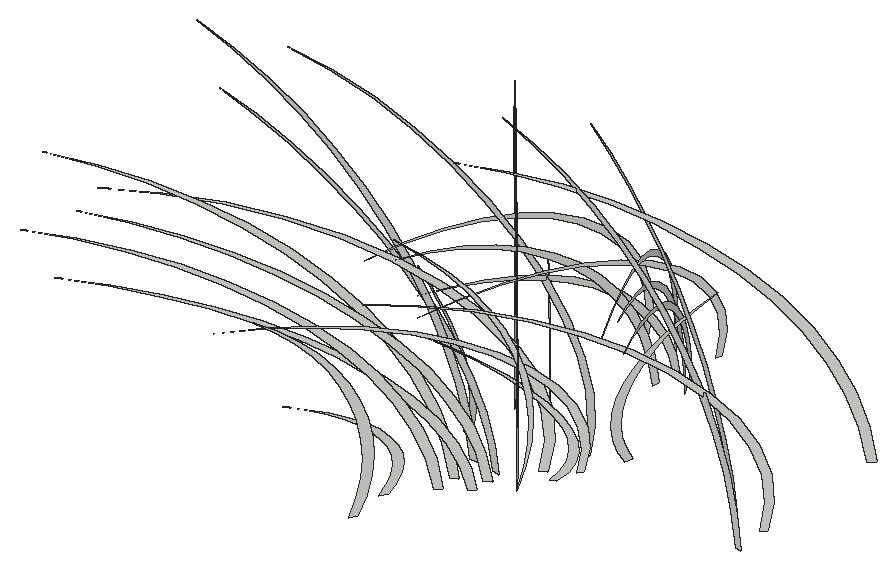
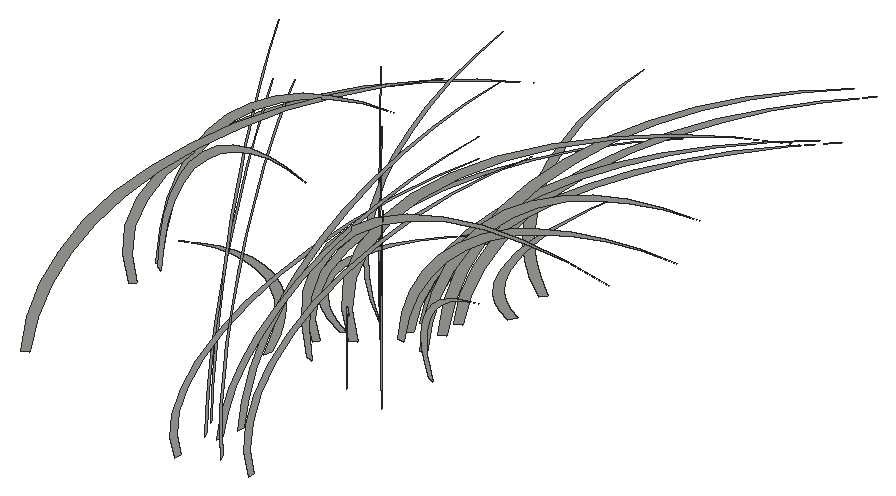
# SketchUp Ruby script. Lengths in inches.
U = 1.inch
M = Sketchup.active_model
def pt(a) = Geom::Point3d.new(a.map { |v| v * U })
def face(e, loops, mat)
  f = e.add_face(loops[0].map { |a| pt(a) })
  loops[1..].each { |l| e.add_face(l.map { |a| pt(a) }).erase! }
  f.material = f.back_material = mat if mat
  f
end
# faces: each face lists its corners as indices into pts; further lists are holes
def faces(e, pts, list, mat = nil) = list.each { |f| face(e, (f[0].is_a?(Array) ? f : [f]).map { |l| l.map { |i| pts[i] } }, mat) }
# xy, xz, yz: faces in a plane at the given z, y or x. An outline is a flat list of corners, or four numbers for a rectangle; further outlines are holes
def ring(l) = l.size == 4 ? [[l[0], l[1]], [l[2], l[1]], [l[2], l[3]], [l[0], l[3]]] : l.each_slice(2).to_a
def flat(e, list, mat, &to3) = list.each { |f| face(e, (f[0].is_a?(Array) ? f : [f]).map { |l| ring(l).map { |u, v| to3.(u, v) } }, mat) }
def xy(e, z, list, mat = nil) = flat(e, list, mat) { |x, y| [x, y, z] }
def xz(e, y, list, mat = nil) = flat(e, list, mat) { |x, z| [x, y, z] }
def yz(e, x, list, mat = nil) = flat(e, list, mat) { |y, z| [x, y, z] }
def lines(e, pts, list) = list.each { |a, b| e.add_line(pt(pts[a]), pt(pts[b])) }
# prism: a flat outline (further loops are holes) pulled along v
def prism(e, loops, v, mat = nil)
  f = face(e, loops, mat); d = Geom::Vector3d.new(v.map { |x| x * U })
  f.pushpull(f.normal.samedirection?(d) ? d.length : -d.length)
end
def box(e, o, s, mat = nil) = prism(e, [[o, [o[0] + s[0], o[1], o[2]], [o[0] + s[0], o[1] + s[1], o[2]], [o[0], o[1] + s[1], o[2]]]], [0, 0, s[2]], mat)
def at(x, y, z, deg = 0) = Geom::Transformation.translation(pt([x, y, z])) * Geom::Transformation.rotation(ORIGIN, Z_AXIS, deg.degrees)
def axes(o, x, y, z) = Geom::Transformation.new([*x, 0, *y, 0, *z, 0, *pt(o).to_a, 1])
def part(name) = M.definitions.add(name)
# library, detail: a bought-in or finely detailed component or shape, given as its bounding box
def library(name, o, s) = part(name).tap { |d| box(d.entities, o, s) }
def detail(e, o, s) = box(e.add_group.entities, o, s)
def put(e, d, t, mat = nil) = e.add_instance(d, t).tap { |i| i.material = mat if mat }
def group(e, t, mat = nil) = e.add_group.tap { |g| g.transformation = t; g.material = mat if mat }.entities
root = M.entities
g1 = group(root,at(13.86,752.1,-58.625))
p = [[-2.41,-3.66,8.31],[-1.97,-2.99,7.78],[-1.57,-2.39,7.2],[-1.22,-1.85,6.58],[-0.92,-1.39,5.92],[-0.67,-1.01,5.22],
  [-0.47,-0.72,4.5],[-0.33,-0.5,3.76],[-0.25,-0.38,3.01],[-0.23,-0.34,2.25],[-0.26,-0.4,1.49],[-0.35,-0.54,0.74],
  [-0.5,-0.77,0],[-0.31,-0.47,0],[-0.14,-0.22,0.75],[-0.04,-0.06,1.51],[0,0,2.29],[-0.03,-0.04,3.0625],
  [-0.12,-0.18,3.83],[-0.27,-0.42,4.58],[-0.49,-0.75,5.31],[-0.77,-1.17,6],[-1.1,-1.68,6.65],[-1.49,-2.27,7.26],
  [-1.93,-2.93,7.82]]
faces(g1,p,[[0,1,2,3,4,5,6,7,8,9,10,11,12,13,14,15,16,17,18,19,20,21,22,23,24]])
g2 = group(root,at(14.625,754.95,-58.625))
p = [[-10.47,-7.14,9.36],[-12.05,-8.22,9.61],[-10.52,-7.17,9.31],[-9.04,-6.16,8.89],[-7.64,-5.2,8.37],[-6.3125,-4.3,7.74],
  [-5.09,-3.47,7.02],[-3.97,-2.71,6.2],[-2.99,-2.04,5.3],[-2.14,-1.46,4.34],[-1.44,-0.98,3.3125],[-0.89,-0.6,2.24],
  [-0.5,-0.34,1.13],[-0.27,-0.1875,0],[0,0,0],[-0.18,-0.125,1.16],[-0.55,-0.375,2.3],[-1.09,-0.74,3.39],
  [-1.8,-1.22,4.44],[-2.66,-1.82,5.43],[-3.68,-2.51,6.34],[-4.83,-3.29,7.15],[-6.1,-4.16,7.875],[-7.48,-5.1,8.49],
  [-8.94,-6.09,8.98]]
faces(g2,p,[[0,1,2,3,4,5,6,7,8,9,10,11,12,13,14,15,16,17,18,19,20,21,22,23,24]])
g3 = group(root,at(15.6,755.62,-58.625))
p = [[-10.47,-7.14,7.55],[-12.05,-8.22,7.75],[-10.52,-7.17,7.51],[-9.04,-6.16,7.17],[-7.64,-5.2,6.75],[-6.3125,-4.3,6.24],
  [-5.09,-3.47,5.66],[-3.97,-2.71,5],[-2.99,-2.04,4.28],[-2.14,-1.46,3.5],[-1.44,-0.98,2.67],[-0.89,-0.6,1.81],
  [-0.5,-0.34,0.91],[-0.27,-0.1875,0],[0,0,0],[-0.18,-0.125,0.93],[-0.55,-0.375,1.85],[-1.09,-0.74,2.74],
  [-1.8,-1.22,3.58],[-2.66,-1.82,4.38],[-3.68,-2.51,5.11],[-4.83,-3.29,5.77],[-6.1,-4.16,6.35],[-7.48,-5.1,6.85],
  [-8.94,-6.09,7.25]]
faces(g3,p,[[0,1,2,3,4,5,6,7,8,9,10,11,12,13,14,15,16,17,18,19,20,21,22,23,24]])
g4 = group(root,at(13.69,753.98,-58.625))
p = [[-2.41,-3.66,4.09],[-1.97,-2.99,3.83],[-1.57,-2.39,3.54],[-1.22,-1.85,3.24],[-0.92,-1.39,2.91],[-0.67,-1.01,2.57],
  [-0.47,-0.72,2.22],[-0.33,-0.5,1.85],[-0.25,-0.38,1.48],[-0.23,-0.34,1.11],[-0.26,-0.4,0.73],[-0.35,-0.54,0.36],
  [-0.5,-0.77,0],[-0.31,-0.47,0],[-0.14,-0.22,0.37],[-0.04,-0.06,0.74],[0,0,1.125],[-0.03,-0.04,1.51],
  [-0.12,-0.18,1.88],[-0.27,-0.42,2.25],[-0.49,-0.75,2.61],[-0.77,-1.17,2.95],[-1.1,-1.68,3.27],[-1.49,-2.27,3.57],
  [-1.93,-2.93,3.84]]
faces(g4,p,[[0,1,2,3,4,5,6,7,8,9,10,11,12,13,14,15,16,17,18,19,20,21,22,23,24]])
g5 = group(root,at(14.6,755.86,-58.625))
p = [[-11.25,-5.83,11.01],[-12.95,-6.71,11.3],[-11.31,-5.86,10.95],[-9.72,-5.04,10.46],[-8.2,-4.25,9.85],[-6.78,-3.51,9.11],
  [-5.46,-2.83,8.25],[-4.27,-2.21,7.29],[-3.21,-1.66,6.24],[-2.3,-1.19,5.1],[-1.54,-0.8,3.9],[-0.95,-0.49,2.64],
  [-0.53,-0.28,1.33],[-0.29,-0.15,0],[0,0,0],[-0.2,-0.1,1.36],[-0.59,-0.31,2.7],[-1.17,-0.61,3.99],
  [-1.93,-1,5.23],[-2.86,-1.48,6.39],[-3.95,-2.05,7.45],[-5.19,-2.69,8.42],[-6.56,-3.4,9.27],[-8.03,-4.16,9.99],
  [-9.61,-4.98,10.57]]
faces(g5,p,[[0,1,2,3,4,5,6,7,8,9,10,11,12,13,14,15,16,17,18,19,20,21,22,23,24]])
g6 = group(root,at(14.6,755.86,-58.625))
p = [[-11.25,-5.83,11.01],[-12.95,-6.71,11.3],[-11.31,-5.86,10.95],[-9.72,-5.04,10.46],[-8.2,-4.25,9.85],[-6.78,-3.51,9.11],
  [-5.46,-2.83,8.25],[-4.27,-2.21,7.29],[-3.21,-1.66,6.24],[-2.3,-1.19,5.1],[-1.54,-0.8,3.9],[-0.95,-0.49,2.64],
  [-0.53,-0.28,1.33],[-0.29,-0.15,0],[0,0,0],[-0.2,-0.1,1.36],[-0.59,-0.31,2.7],[-1.17,-0.61,3.99],
  [-1.93,-1,5.23],[-2.86,-1.48,6.39],[-3.95,-2.05,7.45],[-5.19,-2.69,8.42],[-6.56,-3.4,9.27],[-8.03,-4.16,9.99],
  [-9.61,-4.98,10.57]]
faces(g6,p,[[0,1,2,3,4,5,6,7,8,9,10,11,12,13,14,15,16,17,18,19,20,21,22,23,24]])
g7 = group(root,at(15.65,756.4,-58.625))
p = [[-11.25,-5.83,8.88],[-12.95,-6.71,9.11],[-11.31,-5.86,8.83],[-9.72,-5.04,8.4375],[-8.2,-4.25,7.94],[-6.78,-3.51,7.34],
  [-5.46,-2.83,6.66],[-4.27,-2.21,5.88],[-3.21,-1.66,5.03],[-2.3,-1.19,4.12],[-1.54,-0.8,3.14],[-0.95,-0.49,2.125],
  [-0.53,-0.28,1.07],[-0.29,-0.15,0],[0,0,0],[-0.2,-0.1,1.1],[-0.59,-0.31,2.18],[-1.17,-0.61,3.22],
  [-1.93,-1,4.22],[-2.86,-1.48,5.15],[-3.95,-2.05,6.01],[-5.19,-2.69,6.79],[-6.56,-3.4,7.47],[-8.03,-4.16,8.05],
  [-9.61,-4.98,8.52]]
faces(g7,p,[[0,1,2,3,4,5,6,7,8,9,10,11,12,13,14,15,16,17,18,19,20,21,22,23,24]])
g8 = group(root,at(15.65,756.4,-58.625))
p = [[-11.25,-5.83,8.88],[-12.95,-6.71,9.11],[-11.31,-5.86,8.83],[-9.72,-5.04,8.4375],[-8.2,-4.25,7.94],[-6.78,-3.51,7.34],
  [-5.46,-2.83,6.66],[-4.27,-2.21,5.88],[-3.21,-1.66,5.03],[-2.3,-1.19,4.12],[-1.54,-0.8,3.14],[-0.95,-0.49,2.125],
  [-0.53,-0.28,1.07],[-0.29,-0.15,0],[0,0,0],[-0.2,-0.1,1.1],[-0.59,-0.31,2.18],[-1.17,-0.61,3.22],
  [-1.93,-1,4.22],[-2.86,-1.48,5.15],[-3.95,-2.05,6.01],[-5.19,-2.69,6.79],[-6.56,-3.4,7.47],[-8.03,-4.16,8.05],
  [-9.61,-4.98,8.52]]
faces(g8,p,[[0,1,2,3,4,5,6,7,8,9,10,11,12,13,14,15,16,17,18,19,20,21,22,23,24]])
g9 = group(root,at(17.81,759.07,-58.625))
p = [[-0.31,-0.35,0],[-0.14,-0.15,0],[0,0,0.89],[-0.05,-0.0625,1.79],[-0.3,-0.34,2.67],[-0.73,-0.83,3.51],
  [-1.33,-1.51,4.29],[-2.08,-2.37,4.99],[-2.98,-3.39,5.59],[-3.99,-4.54,6.09],[-5.1,-5.8,6.45],[-6.27,-7.13,6.69],
  [-7.47,-8.5,6.79],[-8.68,-9.88,6.74],[-7.49,-8.53,6.75],[-6.32,-7.19,6.625],[-5.18,-5.9,6.37],[-4.11,-4.68,5.99],
  [-3.13,-3.5625,5.49],[-2.26,-2.58,4.89],[-1.53,-1.74,4.2],[-0.94,-1.07,3.4375],[-0.52,-0.59,2.62],[-0.27,-0.31,1.75],
  [-0.2,-0.22,0.875]]
faces(g9,p,[[0,1,2,3,4,5,6,7,8,9,10,11,12,13,14,15,16,17,18,19,20,21,22,23,24]])
g10 = group(root,at(17.81,759.07,-58.625))
p = [[-0.31,-0.35,0],[-0.14,-0.15,0],[0,0,0.89],[-0.05,-0.0625,1.79],[-0.3,-0.34,2.67],[-0.73,-0.83,3.51],
  [-1.33,-1.51,4.29],[-2.08,-2.37,4.99],[-2.98,-3.39,5.59],[-3.99,-4.54,6.09],[-5.1,-5.8,6.45],[-6.27,-7.13,6.69],
  [-7.47,-8.5,6.79],[-8.68,-9.88,6.74],[-7.49,-8.53,6.75],[-6.32,-7.19,6.625],[-5.18,-5.9,6.37],[-4.11,-4.68,5.99],
  [-3.13,-3.5625,5.49],[-2.26,-2.58,4.89],[-1.53,-1.74,4.2],[-0.94,-1.07,3.4375],[-0.52,-0.59,2.62],[-0.27,-0.31,1.75],
  [-0.2,-0.22,0.875]]
faces(g10,p,[[0,1,2,3,4,5,6,7,8,9,10,11,12,13,14,15,16,17,18,19,20,21,22,23,24]])
g11 = group(root,at(16.94,758.25,-58.625))
p = [[-0.5,-0.26,0],[-0.22,-0.12,0],[0,0,1.26],[-0.09,-0.05,2.52],[-0.49,-0.25,3.76],[-1.19,-0.62,4.94],
  [-2.17,-1.13,6.04],[-3.42,-1.77,7.03],[-4.89,-2.53,7.88],[-6.55,-3.39,8.57],[-8.36,-4.33,9.09],[-10.28,-5.33,9.42],
  [-12.25,-6.35,9.56],[-14.24,-7.38,9.49],[-12.29,-6.37,9.51],[-10.36,-5.37,9.33],[-8.5,-4.41,8.97],[-6.75,-3.5,8.44],
  [-5.14,-2.66,7.74],[-3.71,-1.92,6.89],[-2.51,-1.3,5.92],[-1.55,-0.8,4.84],[-0.85,-0.44,3.68],[-0.44,-0.23,2.47],
  [-0.32,-0.17,1.23]]
faces(g11,p,[[0,1,2,3,4,5,6,7,8,9,10,11,12,13,14,15,16,17,18,19,20,21,22,23,24]])
g12 = group(root,at(17.03,756.92,-58.625))
p = [[-0.32,-0.48,0],[-0.14,-0.22,0.92],[-0.04,-0.05,1.85],[0,0,2.78],[-0.03,-0.05,3.71],[-0.14,-0.21,4.64],
  [-0.32,-0.48,5.5625],[-0.56,-0.85,6.47],[-0.87,-1.33,7.36],[-1.25,-1.9,8.23],[-1.69,-2.58,9.08],[-2.2,-3.35,9.9],
  [-2.77,-4.21,10.69],[-2.23,-3.4,9.89],[-1.76,-2.67,9.0625],[-1.34,-2.03,8.21],[-0.97,-1.48,7.34],[-0.67,-1.02,6.45],
  [-0.43,-0.66,5.54],[-0.26,-0.39,4.625],[-0.14,-0.21,3.7],[-0.09,-0.14,2.78],[-0.1,-0.16,1.85],[-0.18,-0.27,0.92]]
faces(g12,p,[[0,1,2,3,4,5,6,7,8,9,10,11,12,13,14,15,16,17,18,19,20,21,22,23]])
g13 = group(root,at(25.38,759.76,-58.625))
p = [[-0.41,-0.29,0],[-0.18,-0.125,0],[0,0,1.11],[-0.07,-0.05,2.23],[-0.4,-0.28,3.33],[-0.97,-0.68,4.375],
  [-1.78,-1.24,5.35],[-2.79,-1.95,6.22],[-4,-2.79,6.97],[-5.35,-3.73,7.59],[-6.83,-4.77,8.05],[-8.4,-5.86,8.34],
  [-10.02,-6.99,8.46],[-11.64,-8.12,8.4],[-10.05,-7.01,8.41],[-8.47,-5.91,8.26],[-6.95,-4.85,7.9375],[-5.51,-3.85,7.47],
  [-4.2,-2.93,6.85],[-3.04,-2.12,6.1],[-2.05,-1.43,5.24],[-1.26,-0.88,4.28],[-0.7,-0.49,3.26],[-0.36,-0.25,2.1875],
  [-0.26,-0.18,1.09]]
faces(g13,p,[[0,1,2,3,4,5,6,7,8,9,10,11,12,13,14,15,16,17,18,19,20,21,22,23,24]])
g14 = group(root,at(25.38,759.76,-58.625))
p = [[-0.41,-0.29,0],[-0.18,-0.125,0],[0,0,1.11],[-0.07,-0.05,2.23],[-0.4,-0.28,3.33],[-0.97,-0.68,4.375],
  [-1.78,-1.24,5.35],[-2.79,-1.95,6.22],[-4,-2.79,6.97],[-5.35,-3.73,7.59],[-6.83,-4.77,8.05],[-8.4,-5.86,8.34],
  [-10.02,-6.99,8.46],[-11.64,-8.12,8.4],[-10.05,-7.01,8.41],[-8.47,-5.91,8.26],[-6.95,-4.85,7.9375],[-5.51,-3.85,7.47],
  [-4.2,-2.93,6.85],[-3.04,-2.12,6.1],[-2.05,-1.43,5.24],[-1.26,-0.88,4.28],[-0.7,-0.49,3.26],[-0.36,-0.25,2.1875],
  [-0.26,-0.18,1.09]]
faces(g14,p,[[0,1,2,3,4,5,6,7,8,9,10,11,12,13,14,15,16,17,18,19,20,21,22,23,24]])
g15 = group(root,at(18.09,758.06,-58.625))
p = [[-5.5,-1.82,4.81],[-4.45,-1.47,4.5],[-3.51,-1.16,4.17],[-2.67,-0.88,3.81],[-1.95,-0.65,3.43],[-1.36,-0.45,3.02],
  [-0.9,-0.3,2.61],[-0.5625,-0.1875,2.18],[-0.37,-0.12,1.74],[-0.3125,-0.1,1.3],[-0.4,-0.13,0.86],[-0.62,-0.2,0.43],
  [-0.97,-0.32,0],[-0.74,-0.24,0],[-0.33,-0.11,0.42],[-0.07,-0.02,0.86],[0.04,0.01,1.3],[-0.01,0,1.74],
  [-0.21,-0.07,2.18],[-0.5625,-0.1875,2.62],[-1.06,-0.35,3.04],[-1.7,-0.5625,3.44],[-2.47,-0.82,3.83],[-3.37,-1.11,4.18],
  [-4.38,-1.45,4.51]]
faces(g15,p,[[0,1,2,3,4,5,6,7,8,9,10,11,12,13,14,15,16,17,18,19,20,21,22,23,24]])
g16 = group(root,at(17.08,755.99,-58.625))
p = [[-0.37,0.45,0],[-0.16,0.2,1.08],[-0.04,0.05,2.17],[0,0,3.27],[-0.04,0.05,4.37],[-0.16,0.2,5.46],
  [-0.36,0.44,6.54],[-0.65,0.79,7.61],[-1.01,1.23,8.66],[-1.44,1.76,9.6875],[-1.96,2.38,10.6875],[-2.54,3.1,11.65],
  [-3.2,3.9,12.58],[-2.58,3.14,11.64],[-2.03,2.47,10.66],[-1.54,1.88,9.66],[-1.125,1.37,8.63],[-0.78,0.95,7.58],
  [-0.5,0.61,6.52],[-0.29,0.36,5.44],[-0.16,0.2,4.36],[-0.1,0.125,3.27],[-0.12,0.14,2.17],[-0.21,0.25,1.08]]
faces(g16,p,[[0,1,2,3,4,5,6,7,8,9,10,11,12,13,14,15,16,17,18,19,20,21,22,23]])
g17 = group(root,at(15.52,756.9375,-58.625))
p = [[-12.48,2.22,8.88],[-14.36,2.56,9.11],[-12.54,2.23,8.83],[-10.78,1.92,8.4375],[-9.1,1.62,7.94],[-7.52,1.34,7.34],
  [-6.06,1.08,6.66],[-4.74,0.84,5.88],[-3.56,0.63,5.03],[-2.55,0.45,4.12],[-1.71,0.3,3.14],[-1.06,0.1875,2.125],
  [-0.59,0.11,1.07],[-0.33,0.06,0],[0,0,0],[-0.22,0.04,1.1],[-0.65,0.12,2.18],[-1.3,0.23,3.22],
  [-2.14,0.38,4.22],[-3.17,0.57,5.15],[-4.38,0.78,6.01],[-5.76,1.03,6.79],[-7.27,1.3,7.47],[-8.91,1.59,8.05],
  [-10.65,1.9,8.52]]
faces(g17,p,[[0,1,2,3,4,5,6,7,8,9,10,11,12,13,14,15,16,17,18,19,20,21,22,23,24]])
g18 = group(root,at(14.36,757.14,-58.625))
p = [[-12.48,2.22,11.01],[-14.36,2.56,11.3],[-12.54,2.23,10.95],[-10.78,1.92,10.46],[-9.1,1.62,9.85],[-7.52,1.34,9.11],
  [-6.06,1.08,8.25],[-4.74,0.84,7.29],[-3.56,0.63,6.24],[-2.55,0.45,5.1],[-1.71,0.3,3.9],[-1.06,0.1875,2.64],
  [-0.59,0.11,1.33],[-0.33,0.06,0],[0,0,0],[-0.22,0.04,1.36],[-0.65,0.12,2.7],[-1.3,0.23,3.99],
  [-2.14,0.38,5.23],[-3.17,0.57,6.39],[-4.38,0.78,7.45],[-5.76,1.03,8.42],[-7.27,1.3,9.27],[-8.91,1.59,9.99],
  [-10.65,1.9,10.57]]
faces(g18,p,[[0,1,2,3,4,5,6,7,8,9,10,11,12,13,14,15,16,17,18,19,20,21,22,23,24]])
g19 = group(root,at(13.48,758.18,-58.625))
p = [[-3.98,1.82,4.81],[-3.25,1.49,4.5],[-2.6,1.1875,4.17],[-2.02,0.92,3.81],[-1.52,0.69,3.43],[-1.1,0.5,3.02],
  [-0.78,0.36,2.61],[-0.55,0.25,2.18],[-0.41,0.1875,1.74],[-0.375,0.17,1.3],[-0.43,0.2,0.86],[-0.58,0.27,0.43],
  [-0.83,0.38,0],[-0.51,0.23,0],[-0.24,0.11,0.43],[-0.0625,0.03,0.875],[0,0,1.32],[-0.04,0.02,1.77],
  [-0.19,0.09,2.22],[-0.45,0.21,2.65],[-0.8125,0.37,3.07],[-1.27,0.58,3.47],[-1.82,0.84,3.85],[-2.47,1.13,4.2],
  [-3.1875,1.46,4.52]]
faces(g19,p,[[0,1,2,3,4,5,6,7,8,9,10,11,12,13,14,15,16,17,18,19,20,21,22,23,24]])
g20 = group(root,at(25.35,757.96,-58.625))
p = [[-10.97,2.33,11.2],[-12.625,2.68,11.5],[-11.02,2.34,11.14],[-9.47,2.01,10.64],[-8,1.7,10.02],[-6.61,1.41,9.26],
  [-5.33,1.13,8.4],[-4.16,0.88,7.42],[-3.13,0.67,6.35],[-2.24,0.48,5.19],[-1.5,0.32,3.97],[-0.93,0.2,2.68],
  [-0.52,0.11,1.35],[-0.29,0.0625,0],[0,0,0],[-0.19,0.04,1.39],[-0.57,0.12,2.75],[-1.14,0.24,4.0625],
  [-1.88,0.4,5.32],[-2.79,0.59,6.5],[-3.85,0.82,7.58],[-5.06,1.08,8.5625],[-6.39,1.36,9.42],[-7.83,1.67,10.16],
  [-9.37,1.99,10.75]]
faces(g20,p,[[0,1,2,3,4,5,6,7,8,9,10,11,12,13,14,15,16,17,18,19,20,21,22,23,24]])
g21 = group(root,at(15.77,765.41,-58.625))
p = [[-1.83,-10.27,9.0625],[-2.11,-11.82,9.3],[-1.84,-10.32,9.01],[-1.58,-8.87,8.61],[-1.33,-7.49,8.1],[-1.1,-6.1875,7.5],
  [-0.89,-4.99,6.79],[-0.69,-3.9,6],[-0.52,-2.93,5.14],[-0.375,-2.1,4.2],[-0.25,-1.41,3.21],[-0.15,-0.87,2.17],
  [-0.09,-0.49,1.1],[-0.05,-0.27,0],[0,0,0],[-0.03,-0.18,1.12],[-0.1,-0.54,2.22],[-0.19,-1.07,3.29],
  [-0.3125,-1.76,4.3],[-0.47,-2.61,5.26],[-0.64,-3.61,6.13],[-0.84,-4.74,6.93],[-1.07,-5.98,7.625],[-1.31,-7.33,8.22],
  [-1.5625,-8.77,8.7]]
faces(g21,p,[[0,1,2,3,4,5,6,7,8,9,10,11,12,13,14,15,16,17,18,19,20,21,22,23,24]])
g22 = group(root,at(16.05,757.24,-58.625))
p = [[-4.11,5.01,11.96],[-3.46,4.21,11.08],[-2.85,3.47,10.17],[-2.31,2.81,9.23],[-1.82,2.21,8.26],[-1.38,1.68,7.28],
  [-1.01,1.23,6.27],[-0.69,0.85,5.25],[-0.44,0.54,4.21],[-0.25,0.31,3.17],[-0.12,0.15,2.12],[-0.06,0.07,1.06],
  [-0.05,0.07,0],[0,0,1.0625],[-0.02,0.02,2.13],[-0.11,0.14,3.19],[-0.28,0.34,4.25],[-0.52,0.63,5.29],
  [-0.83,1.01,6.32],[-1.21,1.47,7.33],[-1.66,2.02,8.32],[-2.18,2.65,9.28],[-2.76,3.36,10.21],[-3.41,4.15,11.1]]
faces(g22,p,[[0,1,2,3,4,5,6,7,8,9,10,11,12,13,14,15,16,17,18,19,20,21,22,23]])
g23 = group(root,at(16.05,757.24,-58.625))
p = [[-4.11,5.01,11.96],[-3.46,4.21,11.08],[-2.85,3.47,10.17],[-2.31,2.81,9.23],[-1.82,2.21,8.26],[-1.38,1.68,7.28],
  [-1.01,1.23,6.27],[-0.69,0.85,5.25],[-0.44,0.54,4.21],[-0.25,0.31,3.17],[-0.12,0.15,2.12],[-0.06,0.07,1.06],
  [-0.05,0.07,0],[0,0,1.0625],[-0.02,0.02,2.13],[-0.11,0.14,3.19],[-0.28,0.34,4.25],[-0.52,0.63,5.29],
  [-0.83,1.01,6.32],[-1.21,1.47,7.33],[-1.66,2.02,8.32],[-2.18,2.65,9.28],[-2.76,3.36,10.21],[-3.41,4.15,11.1]]
faces(g23,p,[[0,1,2,3,4,5,6,7,8,9,10,11,12,13,14,15,16,17,18,19,20,21,22,23]])
g24 = group(root,at(16.82,765.61,-58.625))
p = [[4.8,-9.26,9.0625],[5.52,-10.66,9.3],[4.82,-9.3,9.01],[4.15,-8,8.61],[3.5,-6.75,8.1],[2.89,-5.58,7.5],
  [2.33,-4.5,6.79],[1.82,-3.51,6],[1.37,-2.64,5.14],[0.98,-1.89,4.2],[0.66,-1.27,3.21],[0.41,-0.78,2.17],
  [0.23,-0.44,1.1],[0.125,-0.24,0],[0,0,0],[0.08,-0.16,1.12],[0.25,-0.49,2.22],[0.5,-0.96,3.29],
  [0.82,-1.59,4.3],[1.22,-2.36,5.26],[1.6875,-3.25,6.13],[2.21,-4.27,6.93],[2.8,-5.4,7.625],[3.43,-6.61,8.22],
  [4.1,-7.91,8.7]]
faces(g24,p,[[0,1,2,3,4,5,6,7,8,9,10,11,12,13,14,15,16,17,18,19,20,21,22,23,24]])
g25 = group(root,at(16.82,765.61,-58.625))
p = [[4.8,-9.26,9.0625],[5.52,-10.66,9.3],[4.82,-9.3,9.01],[4.15,-8,8.61],[3.5,-6.75,8.1],[2.89,-5.58,7.5],
  [2.33,-4.5,6.79],[1.82,-3.51,6],[1.37,-2.64,5.14],[0.98,-1.89,4.2],[0.66,-1.27,3.21],[0.41,-0.78,2.17],
  [0.23,-0.44,1.1],[0.125,-0.24,0],[0,0,0],[0.08,-0.16,1.12],[0.25,-0.49,2.22],[0.5,-0.96,3.29],
  [0.82,-1.59,4.3],[1.22,-2.36,5.26],[1.6875,-3.25,6.13],[2.21,-4.27,6.93],[2.8,-5.4,7.625],[3.43,-6.61,8.22],
  [4.1,-7.91,8.7]]
faces(g25,p,[[0,1,2,3,4,5,6,7,8,9,10,11,12,13,14,15,16,17,18,19,20,21,22,23,24]])
g26 = group(root,at(15.9375,766.37,-58.625))
p = [[-1.83,-10.27,7.31],[-2.11,-11.82,7.5],[-1.84,-10.32,7.27],[-1.58,-8.87,6.94],[-1.33,-7.49,6.54],[-1.1,-6.1875,6.04],
  [-0.89,-4.99,5.48],[-0.69,-3.9,4.84],[-0.52,-2.93,4.14],[-0.375,-2.1,3.39],[-0.25,-1.41,2.59],[-0.15,-0.87,1.75],
  [-0.09,-0.49,0.88],[-0.05,-0.27,0],[0,0,0],[-0.03,-0.18,0.9],[-0.1,-0.54,1.79],[-0.19,-1.07,2.65],
  [-0.3125,-1.76,3.47],[-0.47,-2.61,4.24],[-0.64,-3.61,4.95],[-0.84,-4.74,5.59],[-1.07,-5.98,6.15],[-1.31,-7.33,6.63],
  [-1.5625,-8.77,7.02]]
faces(g26,p,[[0,1,2,3,4,5,6,7,8,9,10,11,12,13,14,15,16,17,18,19,20,21,22,23,24]])
g27 = group(root,at(16.38,766.47,-58.625))
p = [[4.8,-9.26,7.31],[5.52,-10.66,7.5],[4.82,-9.3,7.27],[4.15,-8,6.94],[3.5,-6.75,6.54],[2.89,-5.58,6.04],
  [2.33,-4.5,5.48],[1.82,-3.51,4.84],[1.37,-2.64,4.14],[0.98,-1.89,3.39],[0.66,-1.27,2.59],[0.41,-0.78,1.75],
  [0.23,-0.44,0.88],[0.125,-0.24,0],[0,0,0],[0.08,-0.16,0.9],[0.25,-0.49,1.79],[0.5,-0.96,2.65],
  [0.82,-1.59,3.47],[1.22,-2.36,4.24],[1.6875,-3.25,4.95],[2.21,-4.27,5.59],[2.8,-5.4,6.15],[3.43,-6.61,6.63],
  [4.1,-7.91,7.02]]
faces(g27,p,[[0,1,2,3,4,5,6,7,8,9,10,11,12,13,14,15,16,17,18,19,20,21,22,23,24]])
g28 = group(root,at(16.38,766.47,-58.625))
p = [[4.8,-9.26,7.31],[5.52,-10.66,7.5],[4.82,-9.3,7.27],[4.15,-8,6.94],[3.5,-6.75,6.54],[2.89,-5.58,6.04],
  [2.33,-4.5,5.48],[1.82,-3.51,4.84],[1.37,-2.64,4.14],[0.98,-1.89,3.39],[0.66,-1.27,2.59],[0.41,-0.78,1.75],
  [0.23,-0.44,0.88],[0.125,-0.24,0],[0,0,0],[0.08,-0.16,0.9],[0.25,-0.49,1.79],[0.5,-0.96,2.65],
  [0.82,-1.59,3.47],[1.22,-2.36,4.24],[1.6875,-3.25,4.95],[2.21,-4.27,5.59],[2.8,-5.4,6.15],[3.43,-6.61,6.63],
  [4.1,-7.91,7.02]]
faces(g28,p,[[0,1,2,3,4,5,6,7,8,9,10,11,12,13,14,15,16,17,18,19,20,21,22,23,24]])
g29 = group(root,at(25.1,758.19,-58.625))
p = [[-9.9,5.27,9.74],[-11.4,6.06,10],[-9.95,5.29,9.69],[-8.55,4.55,9.26],[-7.22,3.84,8.71],[-5.97,3.17,8.06],
  [-4.81,2.56,7.3],[-3.76,2,6.45],[-2.83,1.5,5.52],[-2.02,1.08,4.52],[-1.36,0.72,3.45],[-0.84,0.45,2.33],
  [-0.47,0.25,1.18],[-0.26,0.14,0],[0,0,0],[-0.17,0.09,1.21],[-0.52,0.28,2.39],[-1.03,0.55,3.53],
  [-1.7,0.9,4.625],[-2.52,1.34,5.65],[-3.48,1.85,6.6],[-4.57,2.43,7.45],[-5.77,3.07,8.2],[-7.07,3.76,8.84],
  [-8.46,4.5,9.35]]
faces(g29,p,[[0,1,2,3,4,5,6,7,8,9,10,11,12,13,14,15,16,17,18,19,20,21,22,23,24]])
g30 = group(root,at(17.39,759.89,-58.625))
p = [[-0.56,0.1,0],[-0.25,0.04,0],[0,0,1.26],[-0.1,0.02,2.52],[-0.54,0.1,3.76],[-1.32,0.24,4.94],
  [-2.41,0.43,6.04],[-3.79,0.67,7.03],[-5.42,0.97,7.88],[-7.26,1.29,8.57],[-9.27,1.65,9.09],[-11.4,2.03,9.42],
  [-13.59,2.42,9.56],[-15.79,2.8125,9.49],[-13.63,2.43,9.51],[-11.49,2.05,9.33],[-9.43,1.68,8.97],[-7.48,1.33,8.44],
  [-5.7,1.01,7.74],[-4.12,0.73,6.89],[-2.78,0.5,5.92],[-1.71,0.31,4.84],[-0.94,0.17,3.68],[-0.49,0.09,2.47],
  [-0.36,0.0625,1.23]]
faces(g30,p,[[0,1,2,3,4,5,6,7,8,9,10,11,12,13,14,15,16,17,18,19,20,21,22,23,24]])
g31 = group(root,at(17.39,759.89,-58.625))
p = [[-0.56,0.1,0],[-0.25,0.04,0],[0,0,1.26],[-0.1,0.02,2.52],[-0.54,0.1,3.76],[-1.32,0.24,4.94],
  [-2.41,0.43,6.04],[-3.79,0.67,7.03],[-5.42,0.97,7.88],[-7.26,1.29,8.57],[-9.27,1.65,9.09],[-11.4,2.03,9.42],
  [-13.59,2.42,9.56],[-15.79,2.8125,9.49],[-13.63,2.43,9.51],[-11.49,2.05,9.33],[-9.43,1.68,8.97],[-7.48,1.33,8.44],
  [-5.7,1.01,7.74],[-4.12,0.73,6.89],[-2.78,0.5,5.92],[-1.71,0.31,4.84],[-0.94,0.17,3.68],[-0.49,0.09,2.47],
  [-0.36,0.0625,1.23]]
faces(g31,p,[[0,1,2,3,4,5,6,7,8,9,10,11,12,13,14,15,16,17,18,19,20,21,22,23,24]])
g32 = group(root,at(13.51,767.91,-58.625))
p = [[-0.08,-0.46,0],[-0.04,-0.2,0],[0,0,1.03],[-0.01,-0.08,2.07],[-0.08,-0.45,3.09],[-0.19,-1.09,4.07],
  [-0.35,-1.98,4.97],[-0.56,-3.12,5.79],[-0.79,-4.46,6.49],[-1.06,-5.98,7.06],[-1.36,-7.63,7.48],[-1.67,-9.38,7.75],
  [-1.99,-11.18,7.87],[-2.3125,-12.99,7.8125],[-2,-11.22,7.82],[-1.68,-9.46,7.68],[-1.38,-7.76,7.38],[-1.1,-6.16,6.94],
  [-0.84,-4.6875,6.37],[-0.6,-3.39,5.67],[-0.41,-2.29,4.87],[-0.25,-1.41,3.98],[-0.14,-0.78,3.03],[-0.07,-0.4,2.03],
  [-0.05,-0.29,1.02]]
faces(g32,p,[[0,1,2,3,4,5,6,7,8,9,10,11,12,13,14,15,16,17,18,19,20,21,22,23,24]])
g33 = group(root,at(13.51,767.91,-58.625))
p = [[-0.08,-0.46,0],[-0.04,-0.2,0],[0,0,1.03],[-0.01,-0.08,2.07],[-0.08,-0.45,3.09],[-0.19,-1.09,4.07],
  [-0.35,-1.98,4.97],[-0.56,-3.12,5.79],[-0.79,-4.46,6.49],[-1.06,-5.98,7.06],[-1.36,-7.63,7.48],[-1.67,-9.38,7.75],
  [-1.99,-11.18,7.87],[-2.3125,-12.99,7.8125],[-2,-11.22,7.82],[-1.68,-9.46,7.68],[-1.38,-7.76,7.38],[-1.1,-6.16,6.94],
  [-0.84,-4.6875,6.37],[-0.6,-3.39,5.67],[-0.41,-2.29,4.87],[-0.25,-1.41,3.98],[-0.14,-0.78,3.03],[-0.07,-0.4,2.03],
  [-0.05,-0.29,1.02]]
faces(g33,p,[[0,1,2,3,4,5,6,7,8,9,10,11,12,13,14,15,16,17,18,19,20,21,22,23,24]])
g34 = group(root,at(16.32,768.49,-58.625))
p = [[-0.09,-0.49,0],[-0.04,-0.22,0],[0,0,0.88],[-0.02,-0.09,1.76],[-0.09,-0.48,2.63],[-0.21,-1.17,3.46],
  [-0.38,-2.13,4.23],[-0.6,-3.35,4.92],[-0.85,-4.79,5.51],[-1.14,-6.42,6],[-1.46,-8.19,6.36],[-1.79,-10.07,6.59],
  [-2.14,-12,6.6875],[-2.48,-13.95,6.64],[-2.14,-12.04,6.65],[-1.81,-10.15,6.53],[-1.48,-8.33,6.28],[-1.18,-6.61,5.9],
  [-0.9,-5.03,5.41],[-0.65,-3.64,4.82],[-0.4375,-2.46,4.14],[-0.27,-1.51,3.39],[-0.15,-0.83,2.58],[-0.08,-0.43,1.73],
  [-0.06,-0.32,0.86]]
faces(g34,p,[[0,1,2,3,4,5,6,7,8,9,10,11,12,13,14,15,16,17,18,19,20,21,22,23,24]])
g35 = group(root,at(16.32,768.49,-58.625))
p = [[-0.09,-0.49,0],[-0.04,-0.22,0],[0,0,0.88],[-0.02,-0.09,1.76],[-0.09,-0.48,2.63],[-0.21,-1.17,3.46],
  [-0.38,-2.13,4.23],[-0.6,-3.35,4.92],[-0.85,-4.79,5.51],[-1.14,-6.42,6],[-1.46,-8.19,6.36],[-1.79,-10.07,6.59],
  [-2.14,-12,6.6875],[-2.48,-13.95,6.64],[-2.14,-12.04,6.65],[-1.81,-10.15,6.53],[-1.48,-8.33,6.28],[-1.18,-6.61,5.9],
  [-0.9,-5.03,5.41],[-0.65,-3.64,4.82],[-0.4375,-2.46,4.14],[-0.27,-1.51,3.39],[-0.15,-0.83,2.58],[-0.08,-0.43,1.73],
  [-0.06,-0.32,0.86]]
faces(g35,p,[[0,1,2,3,4,5,6,7,8,9,10,11,12,13,14,15,16,17,18,19,20,21,22,23,24]])
g36 = group(root,at(25.1,765.74,-58.625))
p = [[-10.39,-7.25,11.01],[-11.96,-8.35,11.3],[-10.44,-7.29,10.95],[-8.98,-6.26,10.46],[-7.58,-5.29,9.85],[-6.26,-4.37,9.11],
  [-5.05,-3.52,8.25],[-3.94,-2.75,7.29],[-2.97,-2.07,6.24],[-2.12,-1.48,5.1],[-1.42,-0.99,3.9],[-0.88,-0.61,2.64],
  [-0.49,-0.34,1.33],[-0.27,-0.1875,0],[0,0,0],[-0.18,-0.13,1.36],[-0.54,-0.38,2.7],[-1.08,-0.75,3.99],
  [-1.78,-1.24,5.23],[-2.64,-1.84,6.39],[-3.65,-2.55,7.45],[-4.79,-3.34,8.42],[-6.06,-4.23,9.27],[-7.42,-5.18,9.99],
  [-8.875,-6.19,10.57]]
faces(g36,p,[[0,1,2,3,4,5,6,7,8,9,10,11,12,13,14,15,16,17,18,19,20,21,22,23,24]])
g37 = group(root,at(14.86,767.54,-58.625))
p = [[0.21,-0.41,0],[0.09,-0.18,0],[0,0,1.03],[0.04,-0.07,2.07],[0.21,-0.4,3.09],[0.51,-0.98,4.07],
  [0.93,-1.79,4.97],[1.46,-2.8125,5.79],[2.09,-4.02,6.49],[2.79,-5.39,7.06],[3.57,-6.88,7.48],[4.38,-8.46,7.75],
  [5.23,-10.08,7.87],[6.07,-11.72,7.8125],[5.24,-10.11,7.82],[4.42,-8.53,7.68],[3.625,-7,7.38],[2.88,-5.55,6.94],
  [2.19,-4.23,6.37],[1.58,-3.06,5.67],[1.07,-2.0625,4.87],[0.66,-1.27,3.98],[0.36,-0.7,3.03],[0.1875,-0.36,2.03],
  [0.14,-0.27,1.02]]
faces(g37,p,[[0,1,2,3,4,5,6,7,8,9,10,11,12,13,14,15,16,17,18,19,20,21,22,23,24]])
g38 = group(root,at(15.26,760.06,-58.625))
p = [[-2.78,3.38,4.81],[-2.27,2.77,4.5],[-1.8125,2.21,4.17],[-1.41,1.71,3.81],[-1.06,1.29,3.43],[-0.77,0.9375,3.02],
  [-0.54,0.66,2.61],[-0.38,0.47,2.18],[-0.29,0.35,1.74],[-0.26,0.32,1.3],[-0.3,0.37,0.86],[-0.41,0.5,0.43],
  [-0.58,0.71,0],[-0.36,0.4375,0],[-0.16,0.2,0.43],[-0.04,0.05,0.875],[0,0,1.32],[-0.03,0.04,1.77],
  [-0.14,0.17,2.22],[-0.32,0.38,2.65],[-0.57,0.69,3.07],[-0.89,1.08,3.47],[-1.27,1.55,3.85],[-1.72,2.09,4.2],
  [-2.22,2.71,4.52]]
faces(g38,p,[[0,1,2,3,4,5,6,7,8,9,10,11,12,13,14,15,16,17,18,19,20,21,22,23,24]])
g39 = group(root,at(18.125,759.82,-58.625))
p = [[1.43,4.14,5.53],[1.17,3.38,5.18],[0.93,2.7,4.79],[0.72,2.1,4.38],[0.54,1.58,3.9375],[0.39,1.15,3.48],
  [0.28,0.81,3],[0.2,0.57,2.5],[0.15,0.43,2],[0.13,0.39,1.5],[0.15,0.45,0.99],[0.21,0.61,0.49],
  [0.3,0.87,0],[0.18,0.53,0],[0.08,0.25,0.5],[0.02,0.07,1.01],[0,0,1.52],[0.02,0.05,2.04],
  [0.07,0.2,2.55],[0.16,0.47,3.05],[0.29,0.84,3.53],[0.46,1.32,3.99],[0.65,1.9,4.43],[0.88,2.5625,4.83],
  [1.14,3.3125,5.2]]
faces(g39,p,[[0,1,2,3,4,5,6,7,8,9,10,11,12,13,14,15,16,17,18,19,20,21,22,23,24]])
g40 = group(root,at(13.42,760.45,-58.625))
p = [[-2.78,3.38,9.78],[-2.27,2.77,9.15],[-1.8125,2.21,8.47],[-1.41,1.71,7.74],[-1.06,1.29,6.96],[-0.77,0.9375,6.15],
  [-0.54,0.66,5.3],[-0.38,0.47,4.43],[-0.29,0.35,3.54],[-0.26,0.32,2.65],[-0.3,0.37,1.75],[-0.41,0.5,0.87],
  [-0.58,0.71,0],[-0.36,0.4375,0],[-0.16,0.2,0.88],[-0.04,0.05,1.78],[0,0,2.6875],[-0.03,0.04,3.6],
  [-0.14,0.17,4.5],[-0.32,0.38,5.39],[-0.57,0.69,6.24],[-0.89,1.08,7.06],[-1.27,1.55,7.83],[-1.72,2.09,8.54],
  [-2.22,2.71,9.19]]
faces(g40,p,[[0,1,2,3,4,5,6,7,8,9,10,11,12,13,14,15,16,17,18,19,20,21,22,23,24]])
g41 = group(root,at(13.42,760.45,-58.625))
p = [[-2.78,3.38,9.78],[-2.27,2.77,9.15],[-1.8125,2.21,8.47],[-1.41,1.71,7.74],[-1.06,1.29,6.96],[-0.77,0.9375,6.15],
  [-0.54,0.66,5.3],[-0.38,0.47,4.43],[-0.29,0.35,3.54],[-0.26,0.32,2.65],[-0.3,0.37,1.75],[-0.41,0.5,0.87],
  [-0.58,0.71,0],[-0.36,0.4375,0],[-0.16,0.2,0.88],[-0.04,0.05,1.78],[0,0,2.6875],[-0.03,0.04,3.6],
  [-0.14,0.17,4.5],[-0.32,0.38,5.39],[-0.57,0.69,6.24],[-0.89,1.08,7.06],[-1.27,1.55,7.83],[-1.72,2.09,8.54],
  [-2.22,2.71,9.19]]
faces(g41,p,[[0,1,2,3,4,5,6,7,8,9,10,11,12,13,14,15,16,17,18,19,20,21,22,23,24]])
